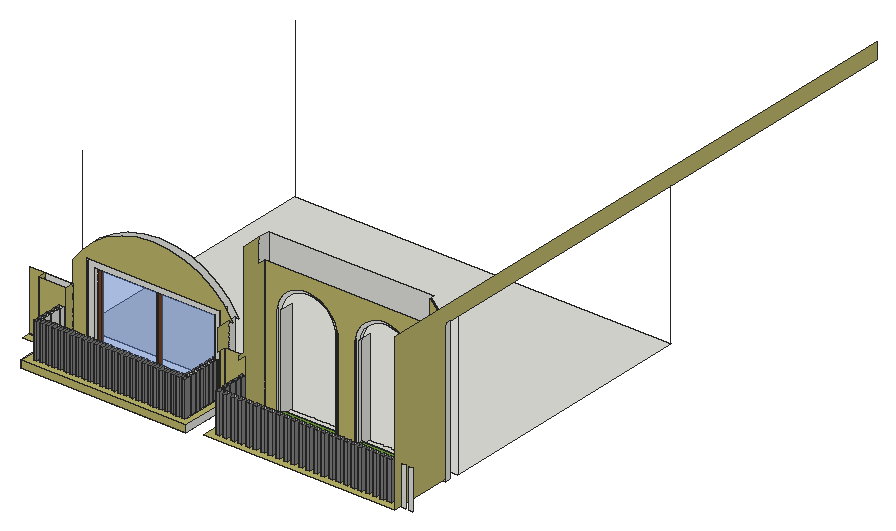
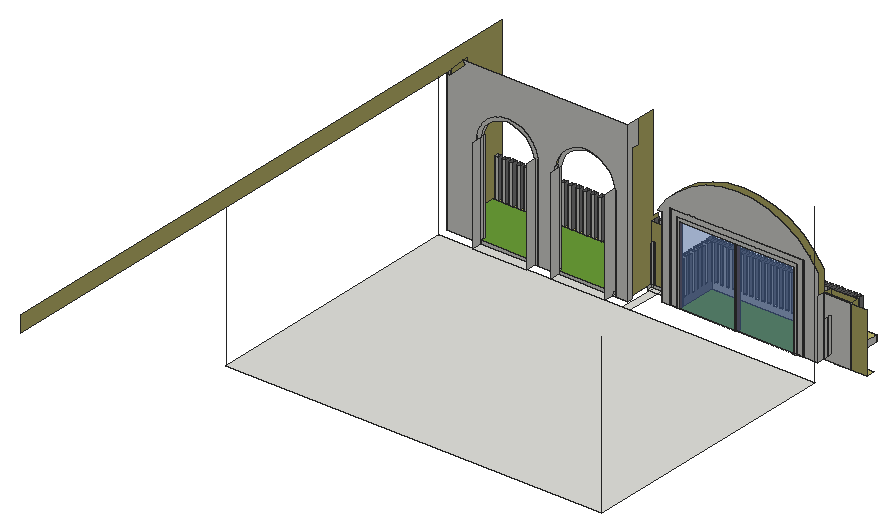
# SketchUp Ruby script. Lengths in inches.
U = 1.inch
M = Sketchup.active_model
def pt(a) = Geom::Point3d.new(a.map { |v| v * U })
def face(e, loops, mat)
  f = e.add_face(loops[0].map { |a| pt(a) })
  loops[1..].each { |l| e.add_face(l.map { |a| pt(a) }).erase! }
  f.material = f.back_material = mat if mat
  f
end
# faces: each face lists its corners as indices into pts; further lists are holes
def faces(e, pts, list, mat = nil) = list.each { |f| face(e, (f[0].is_a?(Array) ? f : [f]).map { |l| l.map { |i| pts[i] } }, mat) }
# xy, xz, yz: faces in a plane at the given z, y or x. An outline is a flat list of corners, or four numbers for a rectangle; further outlines are holes
def ring(l) = l.size == 4 ? [[l[0], l[1]], [l[2], l[1]], [l[2], l[3]], [l[0], l[3]]] : l.each_slice(2).to_a
def flat(e, list, mat, &to3) = list.each { |f| face(e, (f[0].is_a?(Array) ? f : [f]).map { |l| ring(l).map { |u, v| to3.(u, v) } }, mat) }
def xy(e, z, list, mat = nil) = flat(e, list, mat) { |x, y| [x, y, z] }
def xz(e, y, list, mat = nil) = flat(e, list, mat) { |x, z| [x, y, z] }
def yz(e, x, list, mat = nil) = flat(e, list, mat) { |y, z| [x, y, z] }
def lines(e, pts, list) = list.each { |a, b| e.add_line(pt(pts[a]), pt(pts[b])) }
# prism: a flat outline (further loops are holes) pulled along v
def prism(e, loops, v, mat = nil)
  f = face(e, loops, mat); d = Geom::Vector3d.new(v.map { |x| x * U })
  f.pushpull(f.normal.samedirection?(d) ? d.length : -d.length)
end
def box(e, o, s, mat = nil) = prism(e, [[o, [o[0] + s[0], o[1], o[2]], [o[0] + s[0], o[1] + s[1], o[2]], [o[0], o[1] + s[1], o[2]]]], [0, 0, s[2]], mat)
def at(x, y, z, deg = 0) = Geom::Transformation.translation(pt([x, y, z])) * Geom::Transformation.rotation(ORIGIN, Z_AXIS, deg.degrees)
def axes(o, x, y, z) = Geom::Transformation.new([*x, 0, *y, 0, *z, 0, *pt(o).to_a, 1])
def part(name) = M.definitions.add(name)
# library, detail: a bought-in or finely detailed component or shape, given as its bounding box
def library(name, o, s) = part(name).tap { |d| box(d.entities, o, s) }
def detail(e, o, s) = box(e.add_group.entities, o, s)
def put(e, d, t, mat = nil) = e.add_instance(d, t).tap { |i| i.material = mat if mat }
def group(e, t, mat = nil) = e.add_group.tap { |g| g.transformation = t; g.material = mat if mat }.entities
root = M.entities
M.materials.add("[0057_DarkKhaki]").color = [189, 183, 107]
M.materials.add("[0133_Gray]").color = [128, 128, 128]
M.materials.add("[Grass Dark Green]").color = [106, 157, 55]
M.materials.add("[Translucent Glass Blue]").color = [100, 149, 237]
M.materials["[Translucent Glass Blue]"].alpha = 0.5
M.materials.add("[Wood Veneer 01]").color = [120, 70, 37]
xy(root,132,[[54.7,52.4375,54.7,87.625,61.7,87.625,61.7,61.0625,199.44,61.0625,199.44,77.875,205.57,77.875,205.57,52.4375],[61.7,61.0625,194.57,65.0625],[194.57,61.0625,199.44,96.5625],[61.7,65.0625,65.84,87.625],[199.44,77.875,205.57,77.875,205.57,95.25,202.35,95.25,202.35,96.5625,199.44,96.5625],
  [205.57,77.875,205.65,77.875,205.65,90.625,210.07,90.625,210.07,95.25,205.57,95.25],[43.3125,87.625,47.8125,94.9375],[47.8125,87.625,50.0625,90.625],[50.0625,87.625,53.48,94.9375],[53.48,87.625,57.59,90.625],
  [57.59,87.625,68.39,94.9375],[47.8125,90.625,50.0625,94.9375],[53.48,90.625,57.59,94.9375],[210.07,90.625,220.06,94.8125],[220.06,90.625,227.125,94.8125],
  [227.125,90.625,229.2,94.8125],[220.06,94.8125,227.125,125.875],[28.5625,94.9375,43.3125,95.4375],[43.3125,94.9375,47.8125,95.4375],[47.8125,94.9375,50.0625,95.4375],
  [50.0625,94.9375,53.48,95.4375],[53.48,94.9375,57.59,95.4375],[57.59,94.9375,68.39,95.4375],[68.39,95.25,81.22,102.3125],[202.35,95.25,205.57,96.5625],
  [205.57,95.25,210.07,95.25,210.07,102.3125,202.35,102.3125,202.35,96.5625,205.57,96.5625],[229.2,112.125,239.99,116.875],[295.56,112.125,310.99,116.875],[366.56,112.125,394.3125,116.875],[239.99,113.875,242.99,116.875],
  [292.56,113.875,295.56,116.875],[310.99,113.875,313.99,116.875],[363.56,113.875,366.56,116.875],[242.99,116.875,292.56,125.875],[313.99,116.875,363.56,125.875],
  [52.3125,125.875,394.3125,367.8125]])
xy(root,132,[[28.5625,87.625,43.3125,94.9375]],"[0057_DarkKhaki]")
xy(root,132,[[65.84,65.0625,194.57,65.0625,194.57,96.5625,202.35,96.5625,202.35,102.3125,81.22,102.3125,81.22,95.25,68.39,95.25,68.39,87.625,65.84,87.625]],"[Grass Dark Green]")
xy(root,132.08,[[81.29,96.3125,87.22,102.3125],[196.35,96.3125,202.27,102.3125],[141.78,99.3125,143.625,102.3125],[87.22,100.3125,90.22,102.3125],[193.35,100.3125,196.35,102.3125]])
xy(root,134.75,[[226.06,60.1875,226.06,65.875,229.2,65.875,229.2,64.21,229.86,64.21,229.86,60.1875],[232.93,60.1875,236.73,64.21],[239.81,60.1875,243.61,64.21],[246.68,60.1875,250.48,64.21],[253.56,60.1875,257.36,64.21],
  [260.43,60.1875,264.23,64.21],[267.31,60.1875,271.11,64.21],[274.18,60.1875,277.98,64.21],[281.06,60.1875,284.86,64.21],[287.93,60.1875,291.73,64.21],
  [294.81,60.1875,298.61,64.21],[301.68,60.1875,305.48,64.21],[308.56,60.1875,312.36,64.21],[315.43,60.1875,319.23,64.21],[322.31,60.1875,326.11,64.21],
  [329.18,60.1875,332.98,64.21],[336.06,60.1875,339.86,64.21],[342.68,60.1875,346.48,64.21],[349.31,60.1875,353.11,64.21],[355.93,60.1875,359.73,64.21],
  [362.56,60.1875,366.36,64.21],[369.18,60.1875,372.98,64.21],[375.81,60.1875,379.61,64.21],[382.43,60.1875,386.23,64.21],[389.06,60.1875,392.86,64.21],
  [226.06,68.17,229.2,72.0625],[226.06,74.35,229.2,78.25],[226.06,80.54,229.2,84.4375],[226.06,86.73,229.2,90.625],[363.56,112.125,366.56,113.875]])
xy(root,134.75,[[220.06,54.1875,394.3125,54.1875,394.3125,64.21,392.86,64.21,392.86,60.1875,389.06,60.1875,389.06,64.21,386.23,64.21,386.23,60.1875,382.43,60.1875,382.43,64.21,379.61,64.21,379.61,60.1875,375.81,60.1875,375.81,64.21,372.98,64.21,372.98,60.1875,369.18,60.1875,369.18,64.21,366.36,64.21,366.36,60.1875,362.56,60.1875,362.56,64.21,359.73,64.21,359.73,60.1875,355.93,60.1875,355.93,64.21,353.11,64.21,353.11,60.1875,349.31,60.1875,349.31,64.21,346.48,64.21,346.48,60.1875,342.68,60.1875,342.68,64.21,339.86,64.21,339.86,60.1875,336.06,60.1875,336.06,64.21,332.98,64.21,332.98,60.1875,329.18,60.1875,329.18,64.21,326.11,64.21,326.11,60.1875,322.31,60.1875,322.31,64.21,319.23,64.21,319.23,60.1875,315.43,60.1875,315.43,64.21,312.36,64.21,312.36,60.1875,308.56,60.1875,308.56,64.21,305.48,64.21,305.48,60.1875,301.68,60.1875,301.68,64.21,298.61,64.21,298.61,60.1875,294.81,60.1875,294.81,64.21,291.73,64.21,291.73,60.1875,287.93,60.1875,287.93,64.21,284.86,64.21,284.86,60.1875,281.06,60.1875,281.06,64.21,277.98,64.21,277.98,60.1875,274.18,60.1875,274.18,64.21,271.11,64.21,271.11,60.1875,267.31,60.1875,267.31,64.21,264.23,64.21,264.23,60.1875,260.43,60.1875,260.43,64.21,257.36,64.21,257.36,60.1875,253.56,60.1875,253.56,64.21,250.48,64.21,250.48,60.1875,246.68,60.1875,246.68,64.21,243.61,64.21,243.61,60.1875,239.81,60.1875,239.81,64.21,236.73,64.21,236.73,60.1875,232.93,60.1875,232.93,64.21,229.86,64.21,229.86,60.1875,226.06,60.1875,226.06,65.875,229.2,65.875,229.2,68.17,226.06,68.17,226.06,72.0625,229.2,72.0625,229.2,74.35,226.06,74.35,226.06,78.25,229.2,78.25,229.2,80.54,226.06,80.54,226.06,84.4375,229.2,84.4375,229.2,86.73,226.06,86.73,226.06,90.625,220.06,90.625]],"[0057_DarkKhaki]")
xy(root,134.75,[[229.2,64.21,394.3125,64.21,394.3125,112.125,363.56,112.125,363.56,116.875,313.99,116.875,313.99,113.875,310.99,113.875,310.99,112.125,295.56,112.125,295.56,113.875,292.56,113.875,292.56,116.875,242.99,116.875,242.99,113.875,239.99,113.875,239.99,112.125,229.2,112.125]],"[Grass Dark Green]")
xy(root,138.12,[[61.7,59.0625,64.79,61.0625],[67.14,59.0625,70.22,61.0625],[72.57,59.0625,75.66,61.0625],[78.01,59.0625,81.1,61.0625],[83.45,59.0625,86.54,61.0625],
  [88.89,59.0625,91.97,61.0625],[94.32,59.0625,97.41,61.0625],[99.76,59.0625,102.85,61.0625],[105.2,59.0625,108.29,61.0625],[110.64,59.0625,113.72,61.0625],
  [116.07,59.0625,119.16,61.0625],[121.51,59.0625,124.6,61.0625],[126.95,59.0625,130.04,61.0625],[132.39,59.0625,135.47,61.0625],[137.82,59.0625,140.91,61.0625],
  [143.26,59.0625,146.35,61.0625],[148.7,59.0625,151.79,61.0625],[154.14,59.0625,157.22,61.0625],[159.57,59.0625,162.66,61.0625],[165.01,59.0625,168.1,61.0625],
  [170.45,59.0625,173.54,61.0625],[175.64,59.0625,178.72,61.0625],[180.82,59.0625,183.91,61.0625],[186.01,59.0625,189.1,61.0625],[191.2,59.0625,194.29,60.4375],
  [196.39,59.0625,199.44,61.0625],[191.2,60.4375,194.29,61.0625],[64.79,61.0625,67.14,65.0625],[70.22,61.0625,72.57,65.0625],[75.66,61.0625,78.01,65.0625],
  [81.1,61.0625,83.45,65.0625],[86.54,61.0625,88.89,65.0625],[91.97,61.0625,94.32,65.0625],[97.41,61.0625,99.76,65.0625],[102.85,61.0625,105.2,65.0625],
  [108.29,61.0625,110.64,65.0625],[113.72,61.0625,116.07,65.0625],[119.16,61.0625,121.51,65.0625],[124.6,61.0625,126.95,65.0625],[130.04,61.0625,132.39,65.0625],
  [135.47,61.0625,137.82,65.0625],[140.91,61.0625,143.26,65.0625],[146.35,61.0625,148.7,65.0625],[151.79,61.0625,154.14,65.0625],[157.22,61.0625,159.57,65.0625],
  [162.66,61.0625,165.01,65.0625],[168.1,61.0625,170.45,65.0625],[173.54,61.0625,175.64,65.0625],[178.72,61.0625,180.82,65.0625],[183.91,61.0625,186.01,65.0625],
  [189.1,61.0625,191.2,65.0625],[194.29,61.0625,196.39,65.0625],[61.7,62.04,64.79,64.125],[196.39,64.52,199.44,67.1875],[61.7,67.1,65.84,69.1875],
  [194.57,69.52,199.44,72.1875],[61.7,72.16,65.84,74.25],[194.57,74.52,199.44,77.1875],[61.7,77.22,65.84,79.3125],[194.57,79.52,199.44,82.1875],
  [61.7,82.29,65.84,84.375],[194.57,84.52,199.44,87.1875],[194.57,89.52,199.44,92.1875],[194.57,93.58,199.44,96.25]])
xy(root,138.12,[[54.7,52.4375,205.57,52.4375,205.57,96.5625,199.44,96.5625,199.44,59.0625,196.39,59.0625,196.39,61.0625,194.29,61.0625,194.29,59.0625,191.2,59.0625,191.2,61.0625,189.1,61.0625,189.1,59.0625,186.01,59.0625,186.01,61.0625,183.91,61.0625,183.91,59.0625,180.82,59.0625,180.82,61.0625,178.72,61.0625,178.72,59.0625,175.64,59.0625,175.64,61.0625,173.54,61.0625,173.54,59.0625,170.45,59.0625,170.45,61.0625,168.1,61.0625,168.1,59.0625,165.01,59.0625,165.01,61.0625,162.66,61.0625,162.66,59.0625,159.57,59.0625,159.57,61.0625,157.22,61.0625,157.22,59.0625,154.14,59.0625,154.14,61.0625,151.79,61.0625,151.79,59.0625,148.7,59.0625,148.7,61.0625,146.35,61.0625,146.35,59.0625,143.26,59.0625,143.26,61.0625,140.91,61.0625,140.91,59.0625,137.82,59.0625,137.82,61.0625,135.47,61.0625,135.47,59.0625,132.39,59.0625,132.39,61.0625,130.04,61.0625,130.04,59.0625,126.95,59.0625,126.95,61.0625,124.6,61.0625,124.6,59.0625,121.51,59.0625,121.51,61.0625,119.16,61.0625,119.16,59.0625,116.07,59.0625,116.07,61.0625,113.72,61.0625,113.72,59.0625,110.64,59.0625,110.64,61.0625,108.29,61.0625,108.29,59.0625,105.2,59.0625,105.2,61.0625,102.85,61.0625,102.85,59.0625,99.76,59.0625,99.76,61.0625,97.41,61.0625,97.41,59.0625,94.32,59.0625,94.32,61.0625,91.97,61.0625,91.97,59.0625,88.89,59.0625,88.89,61.0625,86.54,61.0625,86.54,59.0625,83.45,59.0625,83.45,61.0625,81.1,61.0625,81.1,59.0625,78.01,59.0625,78.01,61.0625,75.66,61.0625,75.66,59.0625,72.57,59.0625,72.57,61.0625,70.22,61.0625,70.22,59.0625,67.14,59.0625,67.14,61.0625,64.79,61.0625,64.79,59.0625,61.7,59.0625,61.7,87.625,54.7,87.625]],"[0057_DarkKhaki]")
xz(root,52.4375,[[54.7,132,205.57,138.12]],"[0057_DarkKhaki]")
xz(root,59.0625,[[61.7,138.12,64.79,170.16],[67.14,138.12,70.22,170.16],[72.57,138.12,75.66,170.16],[78.01,138.12,81.1,170.16],[83.45,138.12,86.54,170.16],
  [88.89,138.12,91.97,170.16],[94.32,138.12,97.41,170.16],[99.76,138.12,102.85,170.16],[105.2,138.12,108.29,170.16],[110.64,138.12,113.72,170.16],
  [116.07,138.12,119.16,170.16],[121.51,138.12,124.6,170.16],[126.95,138.12,130.04,170.16],[132.39,138.12,135.47,170.16],[137.82,138.12,140.91,170.16],
  [143.26,138.12,146.35,170.16],[148.7,138.12,151.79,170.16],[154.14,138.12,157.22,170.16],[159.57,138.12,162.66,170.16],[165.01,138.12,168.1,170.16],
  [170.45,138.12,173.54,170.16],[175.64,138.12,178.72,170.16],[180.82,138.12,183.91,170.16],[186.01,138.12,189.1,170.16],[191.2,138.12,194.29,170.16],
  [196.39,138.12,199.44,170.16]],"[0133_Gray]")
xz(root,60.1875,[[395.68,134.75,399.48,170.16],[402.31,134.75,406.11,170.16]])
xz(root,60.1875,[[226.06,134.75,229.86,170.16],[232.93,134.75,236.73,170.16],[239.81,134.75,243.61,170.16],[246.68,134.75,250.48,170.16],[253.56,134.75,257.36,170.16],
  [260.43,134.75,264.23,170.16],[267.31,134.75,271.11,170.16],[274.18,134.75,277.98,170.16],[281.06,134.75,284.86,170.16],[287.93,134.75,291.73,170.16],
  [294.81,134.75,298.61,170.16],[301.68,134.75,305.48,170.16],[308.56,134.75,312.36,170.16],[315.43,134.75,319.23,170.16],[322.31,134.75,326.11,170.16],
  [329.18,134.75,332.98,170.16],[336.06,134.75,339.86,170.16],[342.68,134.75,346.48,170.16],[349.31,134.75,353.11,170.16],[355.93,134.75,359.73,170.16],
  [362.56,134.75,366.36,170.16],[369.18,134.75,372.98,170.16],[375.81,134.75,379.61,170.16],[382.43,134.75,386.23,170.16],[389.06,134.75,392.86,170.16]],"[0133_Gray]")
xz(root,61.0625,[[61.7,132,199.44,138.12]])
xz(root,62.04,[[61.7,138.12,64.79,170.16]])
xz(root,64.125,[[61.7,138.12,64.79,170.16]],"[0133_Gray]")
xz(root,64.21,[[229.2,134.75,229.86,170.16],[232.93,134.75,236.73,170.16],[239.81,134.75,243.61,170.16],[246.68,134.75,250.48,170.16],[253.56,134.75,257.36,170.16],
  [260.43,134.75,264.23,170.16],[267.31,134.75,271.11,170.16],[274.18,134.75,277.98,170.16],[281.06,134.75,284.86,170.16],[287.93,134.75,291.73,170.16],
  [294.81,134.75,298.61,170.16],[301.68,134.75,305.48,170.16],[308.56,134.75,312.36,170.16],[315.43,134.75,319.23,170.16],[322.31,134.75,326.11,170.16],
  [329.18,134.75,332.98,170.16],[336.06,134.75,339.86,170.16],[342.68,134.75,346.48,170.16],[349.31,134.75,353.11,170.16],[355.93,134.75,359.73,170.16],
  [362.56,134.75,366.36,170.16],[369.18,134.75,372.98,170.16],[375.81,134.75,379.61,170.16],[382.43,134.75,386.23,170.16],[389.06,134.75,392.86,170.16]])
xz(root,64.52,[[196.39,138.12,199.44,170.16]])
xz(root,65.0625,[[65.84,132,65.84,138.12,67.14,138.12,67.14,170.16,70.22,170.16,70.22,138.12,72.57,138.12,72.57,170.16,75.66,170.16,75.66,138.12,78.01,138.12,78.01,170.16,81.1,170.16,81.1,138.12,83.45,138.12,83.45,170.16,86.54,170.16,86.54,138.12,88.89,138.12,88.89,170.16,91.97,170.16,91.97,138.12,94.32,138.12,94.32,170.16,97.41,170.16,97.41,138.12,99.76,138.12,99.76,170.16,102.85,170.16,102.85,138.12,105.2,138.12,105.2,170.16,108.29,170.16,108.29,138.12,110.64,138.12,110.64,170.16,113.72,170.16,113.72,138.12,116.07,138.12,116.07,170.16,119.16,170.16,119.16,138.12,121.51,138.12,121.51,170.16,124.6,170.16,124.6,138.12,126.95,138.12,126.95,170.16,130.04,170.16,130.04,138.12,132.39,138.12,132.39,170.16,135.47,170.16,135.47,138.12,137.82,138.12,137.82,170.16,140.91,170.16,140.91,138.12,143.26,138.12,143.26,170.16,146.35,170.16,146.35,138.12,148.7,138.12,148.7,170.16,151.79,170.16,151.79,138.12,154.14,138.12,154.14,170.16,157.22,170.16,157.22,138.12,159.57,138.12,159.57,170.16,162.66,170.16,162.66,138.12,165.01,138.12,165.01,170.16,168.1,170.16,168.1,138.12,170.45,138.12,170.45,170.16,173.54,170.16,173.54,138.12,175.64,138.12,175.64,170.16,178.72,170.16,178.72,138.12,180.82,138.12,180.82,170.16,183.91,170.16,183.91,138.12,186.01,138.12,186.01,170.16,189.1,170.16,189.1,138.12,191.2,138.12,191.2,170.16,194.29,170.16,194.29,138.12,194.57,138.12,194.57,132],[64.79,138.12,65.84,170.16],[65.84,138.12,67.14,170.16]])
xz(root,65.0625,[[194.57,138.12,196.39,170.16]],"[0133_Gray]")
xz(root,65.875,[[226.06,134.75,229.2,170.16]])
xz(root,67.1,[[61.7,138.12,65.84,170.16]])
xz(root,67.1875,[[196.39,138.12,199.44,170.16]],"[0133_Gray]")
xz(root,68.17,[[226.06,134.75,229.2,170.16]],"[0133_Gray]")
xz(root,69.1875,[[61.7,138.12,65.84,170.16]],"[0133_Gray]")
xz(root,69.52,[[194.57,138.12,199.44,170.16]])
xz(root,72.0625,[[226.06,134.75,229.2,170.16]])
xz(root,72.16,[[61.7,138.12,65.84,170.16]])
xz(root,72.1875,[[194.57,138.12,199.44,170.16]],"[0133_Gray]")
xz(root,74.25,[[61.7,138.12,65.84,170.16]],"[0133_Gray]")
xz(root,74.35,[[226.06,134.75,229.2,170.16]],"[0133_Gray]")
xz(root,74.52,[[194.57,138.12,199.44,170.16]])
xz(root,77.1875,[[194.57,138.12,199.44,170.16]],"[0133_Gray]")
xz(root,77.22,[[61.7,138.12,65.84,170.16]])
xz(root,78.25,[[226.06,134.75,229.2,170.16]])
xz(root,79.3125,[[61.7,138.12,65.84,170.16]],"[0133_Gray]")
xz(root,79.52,[[194.57,138.12,199.44,170.16]])
xz(root,80.54,[[226.06,134.75,229.2,170.16]],"[0133_Gray]")
xz(root,82.1875,[[194.57,138.12,199.44,170.16]],"[0133_Gray]")
xz(root,82.29,[[61.7,138.12,65.84,170.16]])
xz(root,84.375,[[61.7,138.12,65.84,170.16]],"[0133_Gray]")
xz(root,84.4375,[[226.06,134.75,229.2,170.16]])
xz(root,84.52,[[194.57,138.12,199.44,170.16]])
xz(root,86.73,[[226.06,134.75,229.2,170.16]],"[0133_Gray]")
xz(root,87.1875,[[194.57,138.12,199.44,170.16]],"[0133_Gray]")
xz(root,87.625,[[54.7,132,61.7,138.12],[61.7,132,65.84,170.16]])
xz(root,87.625,[[43.3125,132,54.7,132,54.7,138.12,61.7,138.12,61.7,170.16,65.84,170.16,65.84,132,68.39,132,68.39,186.28,43.3125,186.28]],"[0057_DarkKhaki]")
xz(root,89.52,[[194.57,138.12,199.44,170.16]])
xz(root,90.625,[[220.06,132,227.125,134.75],[227.125,132,229.2,134.75],[226.06,134.75,227.125,170.16],[227.125,134.75,229.2,170.16]])
xz(root,90.625,[[210.07,132,220.06,132,220.06,134.75,226.06,134.75,226.06,170.16,229.2,170.16,229.2,186.28,210.07,186.28]],"[0057_DarkKhaki]")
xz(root,92.1875,[[194.57,138.12,199.44,170.16]],"[0133_Gray]")
xz(root,93.58,[[194.57,138.12,199.44,170.16]])
xz(root,94.9375,[[43.3125,132,68.39,186.28]])
xz(root,95.25,[[68.39,132,81.22,132,81.22,211.75,202.35,211.75,202.35,132,210.07,132,210.07,205.78,214.14,205.78,205.45,217.36,194.95,227.33,182.92,235.38,169.71,241.31,155.6875,244.93,141.26,246.15,126.83,244.93,112.82,241.31,99.61,235.38,87.58,227.33,77.07,217.36,68.39,205.78]],"[0057_DarkKhaki]")
xz(root,95.4375,[[43.3125,132,68.39,186.28]])
xz(root,95.4375,[[28.5625,132,43.3125,186.28]],"[0057_DarkKhaki]")
xz(root,96.25,[[194.57,138.12,199.44,170.16]])
xz(root,96.3125,[[81.29,132.08,87.22,132.08,87.22,205.75,196.35,205.75,196.35,132.08,202.27,132.08,202.27,211.67,81.29,211.67]])
xz(root,96.5625,[[194.57,132,199.44,170.16],[199.44,132,205.57,138.12]])
xz(root,99.3125,[[141.78,132.08,143.625,202.75]],"[Wood Veneer 01]")
xz(root,100.3125,[[87.22,132.08,90.22,132.08,90.22,202.75,193.35,202.75,193.35,132.08,196.35,132.08,196.35,205.75,87.22,205.75]],"[Wood Veneer 01]")
xz(root,102.3125,[[68.39,132,68.39,205.78,77.07,217.36,87.58,227.33,99.61,235.38,112.82,241.31,126.83,244.93,141.26,246.15,155.6875,244.93,169.71,241.31,182.92,235.38,194.95,227.33,205.45,217.36,214.14,205.78,210.07,205.78,210.07,132,202.35,132,202.35,211.75,81.22,211.75,81.22,132],[81.22,132,87.22,132,87.22,132.08,81.29,132.08,81.29,211.67,202.27,211.67,202.27,132.08,143.625,132.08,143.625,132,202.35,132,202.35,211.75,81.22,211.75],[87.22,132,90.22,132.08],[90.22,132,141.78,132.08],[141.78,132,143.625,132.08],
  [81.29,132.08,81.29,211.67,202.27,211.67,202.27,132.08,196.35,132.08,196.35,205.75,87.22,205.75,87.22,132.08],[87.22,132.08,87.22,205.75,196.35,205.75,196.35,132.08,193.35,132.08,193.35,202.75,90.22,202.75,90.22,132.08],[141.78,132.08,143.625,202.75]])
xz(root,102.3125,[[90.22,132.08,141.78,202.75],[143.625,132.08,193.35,202.75]],"[Translucent Glass Blue]")
xz(root,112.125,[[229.2,132,239.99,134.75],[295.56,132,310.99,134.75],[366.56,132,394.3125,134.75]])
xz(root,112.125,[[229.2,134.75,239.99,134.75,239.99,218.72,241.77,225.16,244.99,230.95,249.47,235.84,254.98,239.53,261.19,241.83,267.77,242.62,274.36,241.83,280.57,239.53,286.08,235.84,290.56,230.95,293.77,225.16,295.56,218.72,295.56,134.75,310.99,134.75,310.99,218.72,312.77,225.16,315.99,230.95,320.47,235.84,325.98,239.53,332.19,241.83,338.77,242.62,345.36,241.83,351.57,239.53,357.08,235.84,361.56,230.95,364.77,225.16,366.56,218.72,363.56,218.72,363.56,134.75,394.3125,134.75,394.3125,261.1,379.41,276,379.33,276,379.33,255,229.2,255]],"[0057_DarkKhaki]")
xz(root,113.875,[[239.99,132,242.99,134.75],[292.56,132,295.56,134.75],[310.99,132,313.99,134.75],[363.56,132,366.56,134.75],[239.99,134.75,242.99,134.75,242.99,218.3125,244.57,224.01,247.44,229.1875,251.44,233.54,256.35,236.84,261.9,238.9,267.77,239.59,273.65,238.9,279.2,236.84,284.11,233.54,288.11,229.1875,290.98,224.01,292.56,218.3125,292.56,134.75,295.56,134.75,295.56,218.72,293.77,225.16,290.56,230.95,286.08,235.84,280.57,239.53,274.36,241.83,267.77,242.62,261.19,241.83,254.98,239.53,249.47,235.84,244.99,230.95,241.77,225.16,239.99,218.72],
  [310.99,134.75,313.99,134.75,313.99,218.3125,315.57,224.01,318.44,229.1875,322.44,233.54,327.35,236.84,332.9,238.9,338.77,239.59,344.65,238.9,350.2,236.84,355.11,233.54,359.11,229.1875,361.98,224.01,363.56,218.3125,363.56,218.72,366.56,218.72,364.77,225.16,361.56,230.95,357.08,235.84,351.57,239.53,345.36,241.83,338.77,242.62,332.19,241.83,325.98,239.53,320.47,235.84,315.99,230.95,312.77,225.16,310.99,218.72],[363.56,134.75,366.56,218.72]])
xz(root,116.875,[[229.2,132,229.2,276,379.41,276,376.8,273.39,391.71,258.49,394.3125,261.1,394.3125,132,366.56,132,366.56,218.72,364.77,225.16,361.56,230.95,357.08,235.84,351.57,239.53,345.36,241.83,338.77,242.62,332.19,241.83,325.98,239.53,320.47,235.84,315.99,230.95,312.77,225.16,310.99,218.72,310.99,132,295.56,132,295.56,218.72,293.77,225.16,290.56,230.95,286.08,235.84,280.57,239.53,274.36,241.83,267.77,242.62,261.19,241.83,254.98,239.53,249.47,235.84,244.99,230.95,241.77,225.16,239.99,218.72,239.99,132],[242.99,132,292.56,134.75],[310.99,132,310.99,218.72,312.77,225.16,315.99,230.95,320.47,235.84,325.98,239.53,332.19,241.83,338.77,242.62,345.36,241.83,351.57,239.53,357.08,235.84,361.56,230.95,364.77,225.16,366.56,218.72,366.56,132,363.56,132,363.56,218.3125,361.98,224.01,359.11,229.1875,355.11,233.54,350.2,236.84,344.65,238.9,338.77,239.59,332.9,238.9,327.35,236.84,322.44,233.54,318.44,229.1875,315.57,224.01,313.99,218.3125,313.99,132],[313.99,132,363.56,134.75]])
yz(root,43.3125,[[94.9375,132,95.4375,186.28]])
yz(root,43.3125,[[87.625,132,94.9375,186.28]],"[0057_DarkKhaki]")
yz(root,54.7,[[52.4375,132,87.625,138.12]])
yz(root,61.7,[[61.0625,132,87.625,138.12],[87.35,138.12,87.625,170.16],[89.4375,138.12,92.41,170.16],[94.5,138.12,97.47,170.16],[99.5625,138.12,102.54,170.16]])
yz(root,61.7,[[59.0625,138.12,62.04,170.16],[64.125,138.12,67.1,170.16],[69.1875,138.12,72.16,170.16],[74.25,138.12,77.22,170.16],[79.3125,138.12,82.29,170.16],
  [84.375,138.12,87.35,170.16]],"[0133_Gray]")
yz(root,64.79,[[64.125,138.12,65.0625,170.16]])
yz(root,64.79,[[59.0625,138.12,62.04,170.16]],"[0133_Gray]")
yz(root,65.84,[[65.0625,132,87.625,132,87.625,170.16,84.375,170.16,84.375,138.12,82.29,138.12,82.29,170.16,79.3125,170.16,79.3125,138.12,77.22,138.12,77.22,170.16,74.25,170.16,74.25,138.12,72.16,138.12,72.16,170.16,69.1875,170.16,69.1875,138.12,67.1,138.12,67.1,170.16,65.0625,170.16]])
yz(root,67.14,[[59.0625,138.12,65.0625,170.16]],"[0133_Gray]")
yz(root,68.39,[[94.9375,132,95.25,186.28],[95.25,132,95.4375,186.28],[95.4375,132,102.3125,186.28]])
yz(root,68.39,[[87.625,132,94.9375,186.28]],"[0057_DarkKhaki]")
yz(root,70.22,[[59.0625,138.12,65.0625,170.16]],"[0133_Gray]")
yz(root,72.57,[[59.0625,138.12,65.0625,170.16]],"[0133_Gray]")
yz(root,75.66,[[59.0625,138.12,65.0625,170.16]],"[0133_Gray]")
yz(root,78.01,[[59.0625,138.12,65.0625,170.16]],"[0133_Gray]")
yz(root,81.1,[[59.0625,138.12,65.0625,170.16]],"[0133_Gray]")
yz(root,81.22,[[95.25,132,102.3125,211.75]])
yz(root,81.29,[[96.3125,132.08,102.3125,211.67]])
yz(root,83.45,[[59.0625,138.12,65.0625,170.16]],"[0133_Gray]")
yz(root,86.54,[[59.0625,138.12,65.0625,170.16]],"[0133_Gray]")
yz(root,87.22,[[96.3125,132.08,100.3125,205.75],[100.3125,132.08,102.3125,205.75]])
yz(root,88.89,[[59.0625,138.12,65.0625,170.16]],"[0133_Gray]")
yz(root,90.22,[[100.3125,132.08,102.3125,202.75]],"[Wood Veneer 01]")
yz(root,91.97,[[59.0625,138.12,65.0625,170.16]],"[0133_Gray]")
yz(root,94.32,[[59.0625,138.12,65.0625,170.16]],"[0133_Gray]")
yz(root,97.41,[[59.0625,138.12,65.0625,170.16]],"[0133_Gray]")
yz(root,99.76,[[59.0625,138.12,65.0625,170.16]],"[0133_Gray]")
yz(root,102.85,[[59.0625,138.12,65.0625,170.16]],"[0133_Gray]")
yz(root,105.2,[[59.0625,138.12,65.0625,170.16]],"[0133_Gray]")
yz(root,108.29,[[59.0625,138.12,65.0625,170.16]],"[0133_Gray]")
yz(root,110.64,[[59.0625,138.12,65.0625,170.16]],"[0133_Gray]")
yz(root,113.72,[[59.0625,138.12,65.0625,170.16]],"[0133_Gray]")
yz(root,116.07,[[59.0625,138.12,65.0625,170.16]],"[0133_Gray]")
yz(root,119.16,[[59.0625,138.12,65.0625,170.16]],"[0133_Gray]")
yz(root,121.51,[[59.0625,138.12,65.0625,170.16]],"[0133_Gray]")
yz(root,124.6,[[59.0625,138.12,65.0625,170.16]],"[0133_Gray]")
yz(root,126.95,[[59.0625,138.12,65.0625,170.16]],"[0133_Gray]")
yz(root,130.04,[[59.0625,138.12,65.0625,170.16]],"[0133_Gray]")
yz(root,132.39,[[59.0625,138.12,65.0625,170.16]],"[0133_Gray]")
yz(root,135.47,[[59.0625,138.12,65.0625,170.16]],"[0133_Gray]")
yz(root,137.82,[[59.0625,138.12,65.0625,170.16]],"[0133_Gray]")
yz(root,140.91,[[59.0625,138.12,65.0625,170.16]],"[0133_Gray]")
yz(root,141.78,[[99.3125,132.08,102.3125,202.75]],"[Wood Veneer 01]")
yz(root,143.26,[[59.0625,138.12,65.0625,170.16]],"[0133_Gray]")
yz(root,143.625,[[99.3125,132.08,102.3125,202.75]],"[Wood Veneer 01]")
yz(root,146.35,[[59.0625,138.12,65.0625,170.16]],"[0133_Gray]")
yz(root,148.7,[[59.0625,138.12,65.0625,170.16]],"[0133_Gray]")
yz(root,151.79,[[59.0625,138.12,65.0625,170.16]],"[0133_Gray]")
yz(root,154.14,[[59.0625,138.12,65.0625,170.16]],"[0133_Gray]")
yz(root,157.22,[[59.0625,138.12,65.0625,170.16]],"[0133_Gray]")
yz(root,159.57,[[59.0625,138.12,65.0625,170.16]],"[0133_Gray]")
yz(root,162.66,[[59.0625,138.12,65.0625,170.16]],"[0133_Gray]")
yz(root,165.01,[[59.0625,138.12,65.0625,170.16]],"[0133_Gray]")
yz(root,168.1,[[59.0625,138.12,65.0625,170.16]],"[0133_Gray]")
yz(root,170.45,[[59.0625,138.12,65.0625,170.16]],"[0133_Gray]")
yz(root,173.54,[[59.0625,138.12,65.0625,170.16]],"[0133_Gray]")
yz(root,175.64,[[59.0625,138.12,65.0625,170.16]],"[0133_Gray]")
yz(root,178.72,[[59.0625,138.12,65.0625,170.16]],"[0133_Gray]")
yz(root,180.82,[[59.0625,138.12,65.0625,170.16]],"[0133_Gray]")
yz(root,183.91,[[59.0625,138.12,65.0625,170.16]],"[0133_Gray]")
yz(root,186.01,[[59.0625,138.12,65.0625,170.16]],"[0133_Gray]")
yz(root,189.1,[[59.0625,138.12,65.0625,170.16]],"[0133_Gray]")
yz(root,191.2,[[59.0625,138.12,65.0625,170.16]],"[0133_Gray]")
yz(root,193.35,[[100.3125,132.08,102.3125,202.75]],"[Wood Veneer 01]")
yz(root,194.29,[[59.0625,138.12,65.0625,170.16]],"[0133_Gray]")
yz(root,194.57,[[65.0625,132,65.0625,170.16,69.52,170.16,69.52,138.12,72.1875,138.12,72.1875,170.16,74.52,170.16,74.52,138.12,77.1875,138.12,77.1875,170.16,79.52,170.16,79.52,138.12,82.1875,138.12,82.1875,170.16,84.52,170.16,84.52,138.12,87.1875,138.12,87.1875,170.16,89.52,170.16,89.52,138.12,92.1875,138.12,92.1875,170.16,93.58,170.16,93.58,138.12,96.25,138.12,96.25,170.16,96.5625,170.16,96.5625,132]],"[0133_Gray]")
yz(root,196.35,[[100.3125,132.08,102.3125,205.75]])
yz(root,196.35,[[96.3125,132.08,100.3125,205.75]],"[Wood Veneer 01]")
yz(root,196.39,[[64.52,138.12,65.0625,170.16],[65.0625,138.12,67.1875,170.16]])
yz(root,196.39,[[59.0625,138.12,64.52,170.16]],"[0133_Gray]")
yz(root,199.44,[[61.0625,132,96.5625,138.12],[96.25,138.12,96.5625,170.16]])
yz(root,199.44,[[59.0625,138.12,64.52,170.16],[67.1875,138.12,69.52,170.16],[72.1875,138.12,74.52,170.16],[77.1875,138.12,79.52,170.16],[82.1875,138.12,84.52,170.16],
  [87.1875,138.12,89.52,170.16],[92.1875,138.12,93.58,170.16]],"[0133_Gray]")
yz(root,202.27,[[96.3125,132.08,102.3125,211.67]])
yz(root,202.35,[[95.25,132,102.3125,211.75]])
yz(root,205.57,[[52.4375,132,96.5625,138.12]])
yz(root,210.07,[[95.25,132,102.3125,205.78]])
yz(root,210.07,[[90.625,132,90.625,186.28,82.875,186.28,82.875,205.78,95.25,205.78,95.25,132]],"[0057_DarkKhaki]")
yz(root,226.06,[[60.1875,134.75,61.98,170.16],[61.98,134.75,65.875,170.16],[68.17,134.75,72.0625,170.16],[74.35,134.75,78.25,170.16],[80.54,134.75,84.4375,170.16],
  [86.73,134.75,90.625,170.16]],"[0133_Gray]")
yz(root,229.2,[[90.625,132,94.8125,134.75],[112.125,132,116.875,132,116.875,276,106.125,276,106.125,255,112.125,255]])
yz(root,229.2,[[90.625,134.75,112.125,134.75,112.125,255,106.125,255,106.125,276,88.1875,276,88.1875,189.28,82.875,189.28,82.875,186.28,90.625,186.28]],"[0057_DarkKhaki]")
yz(root,229.2,[[64.21,134.75,65.875,170.16],[68.17,134.75,72.0625,170.16],[74.35,134.75,78.25,170.16],[80.54,134.75,84.4375,170.16],[86.73,134.75,90.625,170.16]],"[0133_Gray]")
yz(root,229.86,[[60.1875,134.75,64.21,170.16]],"[0133_Gray]")
yz(root,232.93,[[60.1875,134.75,64.21,170.16]],"[0133_Gray]")
yz(root,236.73,[[60.1875,134.75,64.21,170.16]],"[0133_Gray]")
yz(root,239.81,[[60.1875,134.75,64.21,170.16]],"[0133_Gray]")
yz(root,239.99,[[112.125,132,113.875,134.75],[113.875,132,116.875,218.72],[112.125,134.75,113.875,218.72]])
yz(root,242.99,[[113.875,132,116.875,134.75],[116.875,132,125.875,132,125.875,218.3125,113.875,218.3125,113.875,134.75,116.875,134.75]])
yz(root,243.61,[[60.1875,134.75,64.21,170.16]],"[0133_Gray]")
yz(root,246.68,[[60.1875,134.75,64.21,170.16]],"[0133_Gray]")
yz(root,250.48,[[60.1875,134.75,64.21,170.16]],"[0133_Gray]")
yz(root,253.56,[[60.1875,134.75,64.21,170.16]],"[0133_Gray]")
yz(root,257.36,[[60.1875,134.75,64.21,170.16]],"[0133_Gray]")
yz(root,260.43,[[60.1875,134.75,64.21,170.16]],"[0133_Gray]")
yz(root,264.23,[[60.1875,134.75,64.21,170.16]],"[0133_Gray]")
yz(root,267.31,[[60.1875,134.75,64.21,170.16]],"[0133_Gray]")
yz(root,271.11,[[60.1875,134.75,64.21,170.16]],"[0133_Gray]")
yz(root,274.18,[[60.1875,134.75,64.21,170.16]],"[0133_Gray]")
yz(root,277.98,[[60.1875,134.75,64.21,170.16]],"[0133_Gray]")
yz(root,281.06,[[60.1875,134.75,64.21,170.16]],"[0133_Gray]")
yz(root,284.86,[[60.1875,134.75,64.21,170.16]],"[0133_Gray]")
yz(root,287.93,[[60.1875,134.75,64.21,170.16]],"[0133_Gray]")
yz(root,291.73,[[60.1875,134.75,64.21,170.16]],"[0133_Gray]")
yz(root,292.56,[[113.875,132,116.875,134.75],[116.875,132,125.875,218.3125],[113.875,134.75,116.875,218.3125]])
yz(root,294.81,[[60.1875,134.75,64.21,170.16]],"[0133_Gray]")
yz(root,295.56,[[112.125,132,113.875,134.75],[113.875,132,116.875,218.72],[112.125,134.75,113.875,218.72]])
yz(root,298.61,[[60.1875,134.75,64.21,170.16]],"[0133_Gray]")
yz(root,301.68,[[60.1875,134.75,64.21,170.16]],"[0133_Gray]")
yz(root,305.48,[[60.1875,134.75,64.21,170.16]],"[0133_Gray]")
yz(root,308.56,[[60.1875,134.75,64.21,170.16]],"[0133_Gray]")
yz(root,310.99,[[112.125,132,113.875,134.75],[113.875,132,116.875,218.72],[112.125,134.75,113.875,218.72]])
yz(root,312.36,[[60.1875,134.75,64.21,170.16]],"[0133_Gray]")
yz(root,313.99,[[113.875,132,116.875,134.75],[116.875,132,125.875,218.3125],[113.875,134.75,116.875,218.3125]])
yz(root,315.43,[[60.1875,134.75,64.21,170.16]],"[0133_Gray]")
yz(root,319.23,[[60.1875,134.75,64.21,170.16]],"[0133_Gray]")
yz(root,322.31,[[60.1875,134.75,64.21,170.16]],"[0133_Gray]")
yz(root,326.11,[[60.1875,134.75,64.21,170.16]],"[0133_Gray]")
yz(root,329.18,[[60.1875,134.75,64.21,170.16]],"[0133_Gray]")
yz(root,332.98,[[60.1875,134.75,64.21,170.16]],"[0133_Gray]")
yz(root,336.06,[[60.1875,134.75,64.21,170.16]],"[0133_Gray]")
yz(root,339.86,[[60.1875,134.75,64.21,170.16]],"[0133_Gray]")
yz(root,342.68,[[60.1875,134.75,64.21,170.16]],"[0133_Gray]")
yz(root,346.48,[[60.1875,134.75,64.21,170.16]],"[0133_Gray]")
yz(root,349.31,[[60.1875,134.75,64.21,170.16]],"[0133_Gray]")
yz(root,353.11,[[60.1875,134.75,64.21,170.16]],"[0133_Gray]")
yz(root,355.93,[[60.1875,134.75,64.21,170.16]],"[0133_Gray]")
yz(root,359.73,[[60.1875,134.75,64.21,170.16]],"[0133_Gray]")
yz(root,362.56,[[60.1875,134.75,64.21,170.16]],"[0133_Gray]")
yz(root,363.56,[[113.875,132,116.875,134.75],[116.875,132,125.875,218.3125],[112.125,134.75,113.875,218.72],[113.875,134.75,116.875,218.3125]])
yz(root,366.36,[[60.1875,134.75,64.21,170.16]],"[0133_Gray]")
yz(root,366.56,[[112.125,132,113.875,134.75],[113.875,132,116.875,218.72]])
yz(root,369.18,[[60.1875,134.75,64.21,170.16]],"[0133_Gray]")
yz(root,372.98,[[60.1875,134.75,64.21,170.16]],"[0133_Gray]")
yz(root,375.81,[[60.1875,134.75,64.21,170.16]],"[0133_Gray]")
yz(root,379.61,[[60.1875,134.75,64.21,170.16]],"[0133_Gray]")
yz(root,382.43,[[60.1875,134.75,64.21,170.16]],"[0133_Gray]")
yz(root,386.23,[[60.1875,134.75,64.21,170.16]],"[0133_Gray]")
yz(root,389.06,[[60.1875,134.75,64.21,170.16]],"[0133_Gray]")
yz(root,392.86,[[60.1875,134.75,64.21,170.16]])
yz(root,394.3125,[[112.125,132,116.875,261.1]])
yz(root,394.3125,[[54.1875,134.75,54.1875,276,601.9375,276,601.9375,261.1,112.125,261.1,112.125,134.75]],"[0057_DarkKhaki]")
p = [[52.3125,125.875,132],[52.3125,125.875,276],[394.3125,125.875,132],[394.3125,125.875,261.1],[52.3125,367.8125,132],[52.3125,367.8125,276],
  [394.3125,367.8125,132],[394.3125,367.8125,261.1],[199.47,61.0625,138.12],[199.44,61.0625,138.12]]
lines(root,p,[[0,1],[2,3],[4,5],[6,7],[8,9]])
